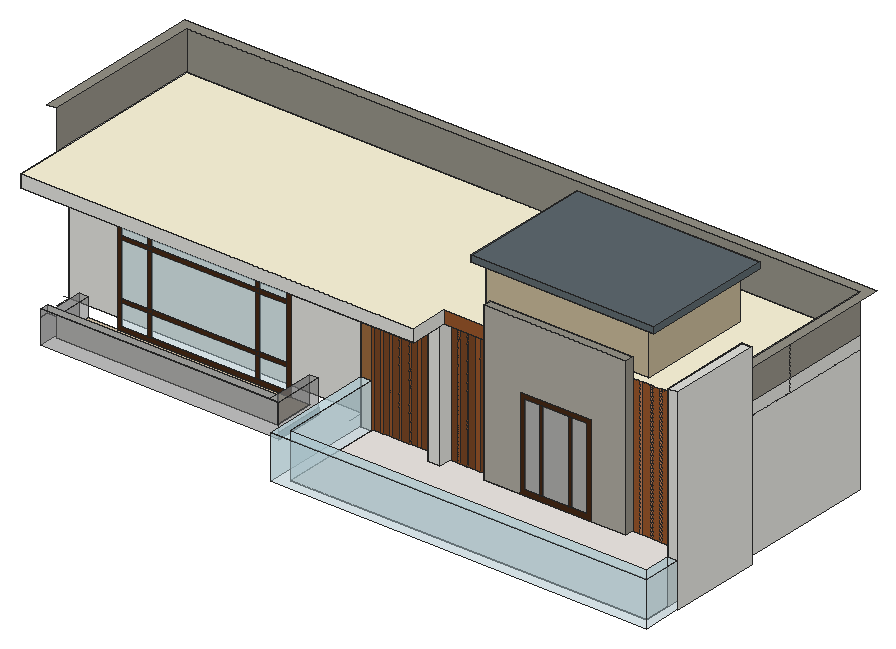
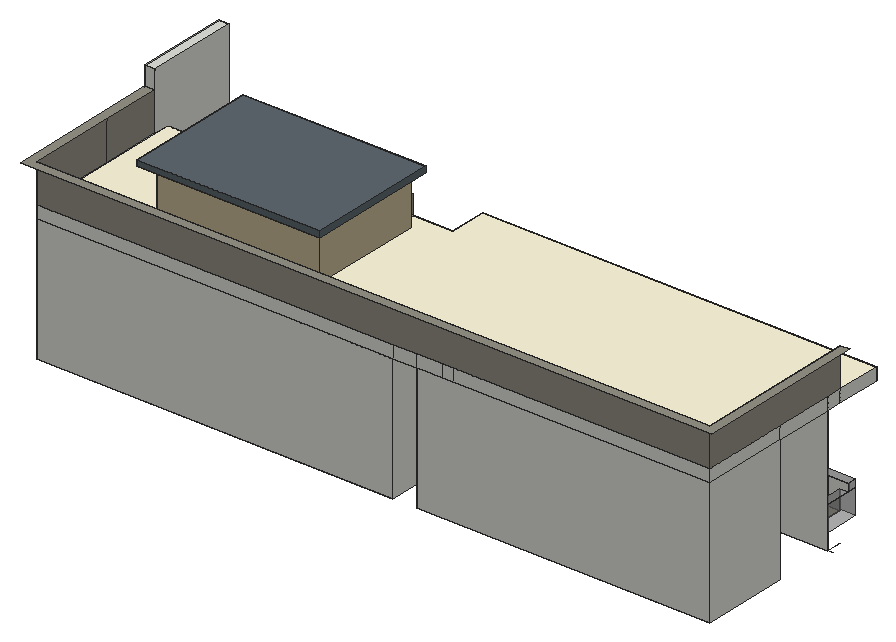
# SketchUp Ruby script. Lengths in inches.
U = 1.inch
M = Sketchup.active_model
def pt(a) = Geom::Point3d.new(a.map { |v| v * U })
def face(e, loops, mat)
  f = e.add_face(loops[0].map { |a| pt(a) })
  loops[1..].each { |l| e.add_face(l.map { |a| pt(a) }).erase! }
  f.material = f.back_material = mat if mat
  f
end
# faces: each face lists its corners as indices into pts; further lists are holes
def faces(e, pts, list, mat = nil) = list.each { |f| face(e, (f[0].is_a?(Array) ? f : [f]).map { |l| l.map { |i| pts[i] } }, mat) }
# xy, xz, yz: faces in a plane at the given z, y or x. An outline is a flat list of corners, or four numbers for a rectangle; further outlines are holes
def ring(l) = l.size == 4 ? [[l[0], l[1]], [l[2], l[1]], [l[2], l[3]], [l[0], l[3]]] : l.each_slice(2).to_a
def flat(e, list, mat, &to3) = list.each { |f| face(e, (f[0].is_a?(Array) ? f : [f]).map { |l| ring(l).map { |u, v| to3.(u, v) } }, mat) }
def xy(e, z, list, mat = nil) = flat(e, list, mat) { |x, y| [x, y, z] }
def xz(e, y, list, mat = nil) = flat(e, list, mat) { |x, z| [x, y, z] }
def yz(e, x, list, mat = nil) = flat(e, list, mat) { |y, z| [x, y, z] }
def lines(e, pts, list) = list.each { |a, b| e.add_line(pt(pts[a]), pt(pts[b])) }
# prism: a flat outline (further loops are holes) pulled along v
def prism(e, loops, v, mat = nil)
  f = face(e, loops, mat); d = Geom::Vector3d.new(v.map { |x| x * U })
  f.pushpull(f.normal.samedirection?(d) ? d.length : -d.length)
end
def box(e, o, s, mat = nil) = prism(e, [[o, [o[0] + s[0], o[1], o[2]], [o[0] + s[0], o[1] + s[1], o[2]], [o[0], o[1] + s[1], o[2]]]], [0, 0, s[2]], mat)
def at(x, y, z, deg = 0) = Geom::Transformation.translation(pt([x, y, z])) * Geom::Transformation.rotation(ORIGIN, Z_AXIS, deg.degrees)
def axes(o, x, y, z) = Geom::Transformation.new([*x, 0, *y, 0, *z, 0, *pt(o).to_a, 1])
def part(name) = M.definitions.add(name)
# library, detail: a bought-in or finely detailed component or shape, given as its bounding box
def library(name, o, s) = part(name).tap { |d| box(d.entities, o, s) }
def detail(e, o, s) = box(e.add_group.entities, o, s)
def put(e, d, t, mat = nil) = e.add_instance(d, t).tap { |i| i.material = mat if mat }
def group(e, t, mat = nil) = e.add_group.tap { |g| g.transformation = t; g.material = mat if mat }.entities
root = M.entities
M.materials.add("[0051_Cornsilk]").color = [255, 248, 220]
M.materials.add("[Color M00]").color = [255, 255, 255]
M.materials.add("[Formica Graystone]").color = [149, 146, 135]
M.materials.add("[Formica Speckled Grey]").color = [94, 105, 111]
M.materials.add("[Quartz Light Brown]").color = [199, 184, 152]
M.materials.add("[Rough Square Concrete Block]").color = [175, 171, 161]
M.materials.add("[Tile Various Tan]").color = [214, 196, 169]
M.materials.add("[Translucent Glass Gray]").color = [128, 128, 128]
M.materials["[Translucent Glass Gray]"].alpha = 0.5
M.materials.add("[Translucent Glass Safety]").color = [204, 235, 244]
M.materials["[Translucent Glass Safety]"].alpha = 0.5
M.materials.add("[Translucent Glass Safety]1").color = [204, 235, 244]
M.materials["[Translucent Glass Safety]1"].alpha = 0.5
M.materials.add("[White Square Tile]").color = [240, 234, 230]
M.materials.add("[Wood Bamboo]").color = [177, 105, 43]
M.materials.add("[Wood Cherry Original]").color = [152, 86, 42]
M.materials.add("[Wood Floor]").color = [155, 105, 61]
M.materials.add("[Wood Veneer 01]").color = [71, 41, 22]
M.materials.add("[Wood Veneer 01]1").color = [120, 70, 37]
M.materials.add("[Wood Veneer 02]").color = [190, 128, 91]
xy(root,141,[[374.25,169.4,386.5,181.59],[424.63,173.96,560.8,181.59],[302.6,179.4,312.93,181.59],[312.93,190.8,653.71,337.49],[9,253.79,289.99,337.49]])
xy(root,141,[[40.13,142.8,251.69,181.59]],"[Tile Various Tan]")
xy(root,141,[[312.93,82.84,653.71,82.84,653.71,181.59,560.8,181.59,560.8,173.96,424.63,173.96,424.63,181.59,386.5,181.59,386.5,169.4,374.25,169.4,374.25,181.59,312.93,181.59]],"[White Square Tile]")
xy(root,159.5,[[31.69,142.8,40.13,181.59]],"[Translucent Glass Gray]")
xy(root,166.97,[[31.69,133.78,251.69,142.8],[251.69,133.78,260.31,181.59]],"[Translucent Glass Gray]")
xy(root,183.75,[[302.6,70.96,662.71,70.96,662.71,108.47,653.71,108.47,653.71,82.84,312.93,82.84,312.93,179.4,302.6,179.4]],"[Translucent Glass Safety]1")
xy(root,261,[[21.23,155.71,20.74,155.74,20.27,155.82,19.8,155.94,19.35,156.11,18.91,156.33,18.51,156.6,18.13,156.9,17.79,157.25,17.48,157.62,17.22,158.03,17,158.46,16.83,158.91,16.7,159.38,16.625,159.86,16.6,160.34,16.625,160.82,16.7,161.3,16.83,161.77,17,162.22,17.22,162.65,17.48,163.06,17.79,163.43,18.13,163.78,18.51,164.08,18.91,164.35,19.35,164.56,19.8,164.74,20.27,164.86,20.74,164.9375,21.23,164.96,21.71,164.9375,22.1875,164.86,22.66,164.74,23.11,164.56,23.54,164.35,23.95,164.08,24.32,163.78,24.66,163.43,24.97,163.06,25.23,162.65,25.45,162.22,25.625,161.77,25.75,161.3,25.83,160.82,25.85,160.34,25.83,159.86,25.75,159.38,25.625,158.91,25.45,158.46,25.23,158.03,24.97,157.62,24.66,157.25,24.32,156.9,23.95,156.6,23.54,156.33,23.11,156.11,22.66,155.94,22.1875,155.82,21.71,155.74],[63.73,155.71,63.24,155.74,62.77,155.82,62.3,155.94,61.85,156.11,61.41,156.33,61.01,156.6,60.63,156.9,60.29,157.25,59.98,157.62,59.72,158.03,59.5,158.46,59.33,158.91,59.2,159.38,59.125,159.86,59.1,160.34,59.125,160.82,59.2,161.3,59.33,161.77,59.5,162.22,59.72,162.65,59.98,163.06,60.29,163.43,60.63,163.78,61.01,164.08,61.41,164.35,61.85,164.56,62.3,164.74,62.77,164.86,63.24,164.9375,63.73,164.96,64.21,164.9375,64.6875,164.86,65.16,164.74,65.61,164.56,66.04,164.35,66.45,164.08,66.82,163.78,67.16,163.43,67.47,163.06,67.73,162.65,67.95,162.22,68.125,161.77,68.25,161.3,68.33,160.82,68.35,160.34,68.33,159.86,68.25,159.38,68.125,158.91,67.95,158.46,67.73,158.03,67.47,157.62,67.16,157.25,66.82,156.9,66.45,156.6,66.04,156.33,65.61,156.11,65.16,155.94,64.6875,155.82,64.21,155.74],[115.79,155.71,115.31,155.74,114.83,155.82,114.36,155.94,113.91,156.11,113.48,156.33,113.07,156.6,112.69,156.9,112.35,157.25,112.05,157.62,111.78,158.03,111.5625,158.46,111.39,158.91,111.27,159.38,111.1875,159.86,111.16,160.34,111.1875,160.82,111.27,161.3,111.39,161.77,111.5625,162.22,111.78,162.65,112.05,163.06,112.35,163.43,112.69,163.78,113.07,164.08,113.48,164.35,113.91,164.56,114.36,164.74,114.83,164.86,115.31,164.9375,115.79,164.96,116.27,164.9375,116.75,164.86,117.22,164.74,117.67,164.56,118.1,164.35,118.51,164.08,118.88,163.78,119.23,163.43,119.53,163.06,119.79,162.65,120.01,162.22,120.1875,161.77,120.3125,161.3,120.39,160.82,120.41,160.34,120.39,159.86,120.3125,159.38,120.1875,158.91,120.01,158.46,119.79,158.03,119.53,157.62,119.23,157.25,118.88,156.9,118.51,156.6,118.1,156.33,117.67,156.11,117.22,155.94,116.75,155.82,116.27,155.74],[172.66,155.71,172.18,155.74,171.7,155.82,171.23,155.94,170.78,156.11,170.35,156.33,169.95,156.6,169.57,156.9,169.23,157.25,168.92,157.62,168.66,158.03,168.4375,158.46,168.27,158.91,168.14,159.38,168.0625,159.86,168.04,160.34,168.0625,160.82,168.14,161.3,168.27,161.77,168.4375,162.22,168.66,162.65,168.92,163.06,169.23,163.43,169.57,163.78,169.95,164.08,170.35,164.35,170.78,164.56,171.23,164.74,171.7,164.86,172.18,164.9375,172.66,164.96,173.15,164.9375,173.625,164.86,174.09,164.74,174.55,164.56,174.98,164.35,175.38,164.08,175.76,163.78,176.1,163.43,176.41,163.06,176.67,162.65,176.89,162.22,177.0625,161.77,177.1875,161.3,177.26,160.82,177.29,160.34,177.26,159.86,177.1875,159.38,177.0625,158.91,176.89,158.46,176.67,158.03,176.41,157.62,176.1,157.25,175.76,156.9,175.38,156.6,174.98,156.33,174.55,156.11,174.09,155.94,173.625,155.82,173.15,155.74],[221.35,155.71,220.87,155.74,220.39,155.82,219.92,155.94,219.47,156.11,219.04,156.33,218.63,156.6,218.26,156.9,217.91,157.25,217.61,157.62,217.35,158.03,217.125,158.46,216.95,158.91,216.83,159.38,216.75,159.86,216.73,160.34,216.75,160.82,216.83,161.3,216.95,161.77,217.125,162.22,217.35,162.65,217.61,163.06,217.91,163.43,218.26,163.78,218.63,164.08,219.04,164.35,219.47,164.56,219.92,164.74,220.39,164.86,220.87,164.9375,221.35,164.96,221.84,164.9375,222.3125,164.86,222.78,164.74,223.23,164.56,223.66,164.35,224.07,164.08,224.45,163.78,224.79,163.43,225.09,163.06,225.36,162.65,225.58,162.22,225.75,161.77,225.875,161.3,225.95,160.82,225.98,160.34,225.95,159.86,225.875,159.38,225.75,158.91,225.58,158.46,225.36,158.03,225.09,157.62,224.79,157.25,224.45,156.9,224.07,156.6,223.66,156.33,223.23,156.11,222.78,155.94,222.3125,155.82,221.84,155.74],
  [280.54,155.71,280.06,155.74,279.58,155.82,279.11,155.94,278.66,156.11,278.23,156.33,277.82,156.6,277.44,156.9,277.1,157.25,276.8,157.62,276.53,158.03,276.3125,158.46,276.14,158.91,276.02,159.38,275.9375,159.86,275.91,160.34,275.9375,160.82,276.02,161.3,276.14,161.77,276.3125,162.22,276.53,162.65,276.8,163.06,277.1,163.43,277.44,163.78,277.82,164.08,278.23,164.35,278.66,164.56,279.11,164.74,279.58,164.86,280.06,164.9375,280.54,164.96,281.02,164.9375,281.5,164.86,281.97,164.74,282.42,164.56,282.85,164.35,283.26,164.08,283.63,163.78,283.98,163.43,284.28,163.06,284.54,162.65,284.76,162.22,284.9375,161.77,285.0625,161.3,285.14,160.82,285.16,160.34,285.14,159.86,285.0625,159.38,284.9375,158.91,284.76,158.46,284.54,158.03,284.28,157.62,283.98,157.25,283.63,156.9,283.26,156.6,282.85,156.33,282.42,156.11,281.97,155.94,281.5,155.82,281.02,155.74],[317.16,155.71,316.68,155.74,316.2,155.82,315.73,155.94,315.28,156.11,314.85,156.33,314.45,156.6,314.07,156.9,313.73,157.25,313.42,157.62,313.16,158.03,312.9375,158.46,312.77,158.91,312.64,159.38,312.5625,159.86,312.54,160.34,312.5625,160.82,312.64,161.3,312.77,161.77,312.9375,162.22,313.16,162.65,313.42,163.06,313.73,163.43,314.07,163.78,314.45,164.08,314.85,164.35,315.28,164.56,315.73,164.74,316.2,164.86,316.68,164.9375,317.16,164.96,317.65,164.9375,318.125,164.86,318.59,164.74,319.05,164.56,319.48,164.35,319.88,164.08,320.26,163.78,320.6,163.43,320.91,163.06,321.17,162.65,321.39,162.22,321.5625,161.77,321.6875,161.3,321.76,160.82,321.79,160.34,321.76,159.86,321.6875,159.38,321.5625,158.91,321.39,158.46,321.17,158.03,320.91,157.62,320.6,157.25,320.26,156.9,319.88,156.6,319.48,156.33,319.05,156.11,318.59,155.94,318.125,155.82,317.65,155.74],[358.29,155.71,357.81,155.74,357.33,155.82,356.86,155.94,356.41,156.11,355.98,156.33,355.57,156.6,355.19,156.9,354.85,157.25,354.55,157.62,354.28,158.03,354.0625,158.46,353.89,158.91,353.77,159.38,353.6875,159.86,353.66,160.34,353.6875,160.82,353.77,161.3,353.89,161.77,354.0625,162.22,354.28,162.65,354.55,163.06,354.85,163.43,355.19,163.78,355.57,164.08,355.98,164.35,356.41,164.56,356.86,164.74,357.33,164.86,357.81,164.9375,358.29,164.96,358.77,164.9375,359.25,164.86,359.72,164.74,360.17,164.56,360.6,164.35,361.01,164.08,361.38,163.78,361.73,163.43,362.03,163.06,362.29,162.65,362.51,162.22,362.6875,161.77,362.8125,161.3,362.89,160.82,362.91,160.34,362.89,159.86,362.8125,159.38,362.6875,158.91,362.51,158.46,362.29,158.03,362.03,157.62,361.73,157.25,361.38,156.9,361.01,156.6,360.6,156.33,360.17,156.11,359.72,155.94,359.25,155.82,358.77,155.74],[374.25,169.4,386.5,181.59],[302.6,179.4,312.93,181.59],
  [312.93,190.8,653.71,196.16],[9,196.16,312.93,253.79],[312.93,196.16,653.71,253.79],[9,253.79,289.99,337.49],[289.99,253.79,312.93,337.49],
  [312.93,253.79,653.71,337.49]])
xy(root,261,[[[9,138.15,9,181.59,302.6,181.59,302.6,179.4,312.93,179.4,312.93,181.59,374.25,181.59,374.25,169.4,386.5,169.4,386.5,138.15],[21.23,155.71,21.71,155.74,22.1875,155.82,22.66,155.94,23.11,156.11,23.54,156.33,23.95,156.6,24.32,156.9,24.66,157.25,24.97,157.62,25.23,158.03,25.45,158.46,25.625,158.91,25.75,159.38,25.83,159.86,25.85,160.34,25.83,160.82,25.75,161.3,25.625,161.77,25.45,162.22,25.23,162.65,24.97,163.06,24.66,163.43,24.32,163.78,23.95,164.08,23.54,164.35,23.11,164.56,22.66,164.74,22.1875,164.86,21.71,164.9375,21.23,164.96,20.74,164.9375,20.27,164.86,19.8,164.74,19.35,164.56,18.91,164.35,18.51,164.08,18.13,163.78,17.79,163.43,17.48,163.06,17.22,162.65,17,162.22,16.83,161.77,16.7,161.3,16.625,160.82,16.6,160.34,16.625,159.86,16.7,159.38,16.83,158.91,17,158.46,17.22,158.03,17.48,157.62,17.79,157.25,18.13,156.9,18.51,156.6,18.91,156.33,19.35,156.11,19.8,155.94,20.27,155.82,20.74,155.74],[317.16,155.71,317.65,155.74,318.125,155.82,318.59,155.94,319.05,156.11,319.48,156.33,319.88,156.6,320.26,156.9,320.6,157.25,320.91,157.62,321.17,158.03,321.39,158.46,321.5625,158.91,321.6875,159.38,321.76,159.86,321.79,160.34,321.76,160.82,321.6875,161.3,321.5625,161.77,321.39,162.22,321.17,162.65,320.91,163.06,320.6,163.43,320.26,163.78,319.88,164.08,319.48,164.35,319.05,164.56,318.59,164.74,318.125,164.86,317.65,164.9375,317.16,164.96,316.68,164.9375,316.2,164.86,315.73,164.74,315.28,164.56,314.85,164.35,314.45,164.08,314.07,163.78,313.73,163.43,313.42,163.06,313.16,162.65,312.9375,162.22,312.77,161.77,312.64,161.3,312.5625,160.82,312.54,160.34,312.5625,159.86,312.64,159.38,312.77,158.91,312.9375,158.46,313.16,158.03,313.42,157.62,313.73,157.25,314.07,156.9,314.45,156.6,314.85,156.33,315.28,156.11,315.73,155.94,316.2,155.82,316.68,155.74],[63.73,155.71,64.21,155.74,64.6875,155.82,65.16,155.94,65.61,156.11,66.04,156.33,66.45,156.6,66.82,156.9,67.16,157.25,67.47,157.62,67.73,158.03,67.95,158.46,68.125,158.91,68.25,159.38,68.33,159.86,68.35,160.34,68.33,160.82,68.25,161.3,68.125,161.77,67.95,162.22,67.73,162.65,67.47,163.06,67.16,163.43,66.82,163.78,66.45,164.08,66.04,164.35,65.61,164.56,65.16,164.74,64.6875,164.86,64.21,164.9375,63.73,164.96,63.24,164.9375,62.77,164.86,62.3,164.74,61.85,164.56,61.41,164.35,61.01,164.08,60.63,163.78,60.29,163.43,59.98,163.06,59.72,162.65,59.5,162.22,59.33,161.77,59.2,161.3,59.125,160.82,59.1,160.34,59.125,159.86,59.2,159.38,59.33,158.91,59.5,158.46,59.72,158.03,59.98,157.62,60.29,157.25,60.63,156.9,61.01,156.6,61.41,156.33,61.85,156.11,62.3,155.94,62.77,155.82,63.24,155.74],[280.54,155.71,281.02,155.74,281.5,155.82,281.97,155.94,282.42,156.11,282.85,156.33,283.26,156.6,283.63,156.9,283.98,157.25,284.28,157.62,284.54,158.03,284.76,158.46,284.9375,158.91,285.0625,159.38,285.14,159.86,285.16,160.34,285.14,160.82,285.0625,161.3,284.9375,161.77,284.76,162.22,284.54,162.65,284.28,163.06,283.98,163.43,283.63,163.78,283.26,164.08,282.85,164.35,282.42,164.56,281.97,164.74,281.5,164.86,281.02,164.9375,280.54,164.96,280.06,164.9375,279.58,164.86,279.11,164.74,278.66,164.56,278.23,164.35,277.82,164.08,277.44,163.78,277.1,163.43,276.8,163.06,276.53,162.65,276.3125,162.22,276.14,161.77,276.02,161.3,275.9375,160.82,275.91,160.34,275.9375,159.86,276.02,159.38,276.14,158.91,276.3125,158.46,276.53,158.03,276.8,157.62,277.1,157.25,277.44,156.9,277.82,156.6,278.23,156.33,278.66,156.11,279.11,155.94,279.58,155.82,280.06,155.74],[115.79,155.71,116.27,155.74,116.75,155.82,117.22,155.94,117.67,156.11,118.1,156.33,118.51,156.6,118.88,156.9,119.23,157.25,119.53,157.62,119.79,158.03,120.01,158.46,120.1875,158.91,120.3125,159.38,120.39,159.86,120.41,160.34,120.39,160.82,120.3125,161.3,120.1875,161.77,120.01,162.22,119.79,162.65,119.53,163.06,119.23,163.43,118.88,163.78,118.51,164.08,118.1,164.35,117.67,164.56,117.22,164.74,116.75,164.86,116.27,164.9375,115.79,164.96,115.31,164.9375,114.83,164.86,114.36,164.74,113.91,164.56,113.48,164.35,113.07,164.08,112.69,163.78,112.35,163.43,112.05,163.06,111.78,162.65,111.5625,162.22,111.39,161.77,111.27,161.3,111.1875,160.82,111.16,160.34,111.1875,159.86,111.27,159.38,111.39,158.91,111.5625,158.46,111.78,158.03,112.05,157.62,112.35,157.25,112.69,156.9,113.07,156.6,113.48,156.33,113.91,156.11,114.36,155.94,114.83,155.82,115.31,155.74],[221.35,155.71,221.84,155.74,222.3125,155.82,222.78,155.94,223.23,156.11,223.66,156.33,224.07,156.6,224.45,156.9,224.79,157.25,225.09,157.62,225.36,158.03,225.58,158.46,225.75,158.91,225.875,159.38,225.95,159.86,225.98,160.34,225.95,160.82,225.875,161.3,225.75,161.77,225.58,162.22,225.36,162.65,225.09,163.06,224.79,163.43,224.45,163.78,224.07,164.08,223.66,164.35,223.23,164.56,222.78,164.74,222.3125,164.86,221.84,164.9375,221.35,164.96,220.87,164.9375,220.39,164.86,219.92,164.74,219.47,164.56,219.04,164.35,218.63,164.08,218.26,163.78,217.91,163.43,217.61,163.06,217.35,162.65,217.125,162.22,216.95,161.77,216.83,161.3,216.75,160.82,216.73,160.34,216.75,159.86,216.83,159.38,216.95,158.91,217.125,158.46,217.35,158.03,217.61,157.62,217.91,157.25,218.26,156.9,218.63,156.6,219.04,156.33,219.47,156.11,219.92,155.94,220.39,155.82,220.87,155.74],[172.66,155.71,173.15,155.74,173.625,155.82,174.09,155.94,174.55,156.11,174.98,156.33,175.38,156.6,175.76,156.9,176.1,157.25,176.41,157.62,176.67,158.03,176.89,158.46,177.0625,158.91,177.1875,159.38,177.26,159.86,177.29,160.34,177.26,160.82,177.1875,161.3,177.0625,161.77,176.89,162.22,176.67,162.65,176.41,163.06,176.1,163.43,175.76,163.78,175.38,164.08,174.98,164.35,174.55,164.56,174.09,164.74,173.625,164.86,173.15,164.9375,172.66,164.96,172.18,164.9375,171.7,164.86,171.23,164.74,170.78,164.56,170.35,164.35,169.95,164.08,169.57,163.78,169.23,163.43,168.92,163.06,168.66,162.65,168.4375,162.22,168.27,161.77,168.14,161.3,168.0625,160.82,168.04,160.34,168.0625,159.86,168.14,159.38,168.27,158.91,168.4375,158.46,168.66,158.03,168.92,157.62,169.23,157.25,169.57,156.9,169.95,156.6,170.35,156.33,170.78,156.11,171.23,155.94,171.7,155.82,172.18,155.74],[358.29,155.71,358.77,155.74,359.25,155.82,359.72,155.94,360.17,156.11,360.6,156.33,361.01,156.6,361.38,156.9,361.73,157.25,362.03,157.62,362.29,158.03,362.51,158.46,362.6875,158.91,362.8125,159.38,362.89,159.86,362.91,160.34,362.89,160.82,362.8125,161.3,362.6875,161.77,362.51,162.22,362.29,162.65,362.03,163.06,361.73,163.43,361.38,163.78,361.01,164.08,360.6,164.35,360.17,164.56,359.72,164.74,359.25,164.86,358.77,164.9375,358.29,164.96,357.81,164.9375,357.33,164.86,356.86,164.74,356.41,164.56,355.98,164.35,355.57,164.08,355.19,163.78,354.85,163.43,354.55,163.06,354.28,162.65,354.0625,162.22,353.89,161.77,353.77,161.3,353.6875,160.82,353.66,160.34,353.6875,159.86,353.77,159.38,353.89,158.91,354.0625,158.46,354.28,158.03,354.55,157.62,354.85,157.25,355.19,156.9,355.57,156.6,355.98,156.33,356.41,156.11,356.86,155.94,357.33,155.82,357.81,155.74]]],"[Wood Bamboo]")
xy(root,261,[[386.5,173.96,424.63,181.59]],"[Wood Cherry Original]")
xy(root,273,[[[9,138.15,386.5,138.15,386.5,173.96,424.63,173.96,424.63,181.59,653.71,181.59,653.71,337.49,9,337.49],[414.15,189.53,570.65,298.28]]],"[0051_Cornsilk]")
xy(root,291,[[424.63,173.96,560.8,181.59]],"[Formica Graystone]")
xy(root,310.4375,[[0,181.59,9,181.59,9,337.49,653.71,337.49,653.71,196.8125,662.71,196.8125,662.71,346.49,0,346.49]],"[Formica Graystone]")
xy(root,318.625,[[407.09,180.78,581.84,189.53],[407.09,189.53,414.15,307.53],[414.15,189.53,570.65,298.28],[570.65,189.53,581.84,307.53],[414.15,298.28,570.65,307.53]])
xy(root,324.375,[[407.09,180.78,581.84,307.53]],"[Formica Speckled Grey]")
xy(root,328.3125,[[653.71,108.47,662.71,196.8125]])
xz(root,70.96,[[302.6,141,662.71,183.75]],"[Translucent Glass Safety]1")
xz(root,82.84,[[312.93,141,653.71,183.75]],"[Translucent Glass Safety]1")
xz(root,108.47,[[653.71,183.75,662.71,328.3125]])
xz(root,133.78,[[31.69,135,260.09,135,260.09,141,260.31,166.97,31.69,166.97]],"[Translucent Glass Gray]")
xz(root,138.15,[[9,261,386.5,273]])
xz(root,142.8,[[40.13,141,40.13,159.5,31.69,159.5,31.69,166.97,251.69,166.97,251.69,141]])
xz(root,169.4,[[374.25,141,386.5,261]])
xz(root,173.96,[[424.63,141,459.54,141,459.54,228.5625,527.66,228.5625,527.66,141,560.8,141,560.8,291,424.63,291]],"[Rough Square Concrete Block]")
xz(root,173.96,[[464.33,145.79,478.25,223.77],[480.65,145.79,506.37,223.77],[508.77,145.79,522.87,223.77]],"[Translucent Glass Gray]")
xz(root,173.96,[[386.5,261,424.63,273]],"[Wood Cherry Original]")
xz(root,173.96,[[[459.54,141,527.66,228.5625],[464.33,145.79,522.87,223.77]],[478.25,145.79,480.65,223.77],[506.37,145.79,508.77,223.77]],"[Wood Veneer 01]")
xz(root,179.4,[[302.6,141,312.93,183.75]])
xz(root,179.4,[[302.6,183.75,312.93,261]],"[Wood Floor]")
xz(root,180.78,[[407.09,318.625,581.84,324.375]],"[Formica Speckled Grey]")
xz(root,181.59,[[302.6,141,312.93,261],[374.25,141,386.5,261],[424.63,141,560.8,261],[424.63,261,560.8,273],[424.63,273,560.8,291]])
xz(root,181.59,[[386.5,141,386.57,261]],"[Color M00]")
xz(root,181.59,[[71.91,145.08,96.9,165.54],[100.71,145.08,199.91,165.54],[203.5,145.08,229.7,165.54],[71.91,169.15,96.9,219.6],[100.71,169.15,199.91,219.6],
  [203.5,169.15,229.7,219.6],[71.91,223.22,96.9,245.05],[100.71,223.22,199.91,245.05],[203.5,223.22,229.7,245.05]],"[Translucent Glass Safety]")
xz(root,181.59,[[319.79,141,321.62,261],[328.48,141,330.5,261],[337.36,141,339.62,261],[346.48,141,348.31,261],[355.17,141,357.85,261],
  [364.71,141,367.39,261],[393.43,141,395.64,261],[402.5,141,403.57,261],[410.43,141,414.51,261],[421.37,141,424.63,261],
  [560.8,141,568.2,273],[570.68,141,578.08,273],[580.05,141,587.45,273],[589.43,141,596.83,273],[598.8,141,606.2,273],
  [608.18,141,615.58,273],[617.55,141,624.95,273],[626.93,141,634.33,273],[636.3,141,643.7,273],[646.31,141,653.71,273]],"[Wood Cherry Original]")
xz(root,181.59,[[[67.84,141,233.77,249.125],[71.91,145.08,229.7,245.05]],[96.9,145.08,100.71,165.54],[199.91,145.08,203.5,165.54],[71.91,165.54,96.9,169.15],[96.9,165.54,100.71,169.15],
  [100.71,165.54,199.91,169.15],[199.91,165.54,203.5,169.15],[203.5,165.54,229.7,169.15],[96.9,169.15,100.71,219.6],[199.91,169.15,203.5,219.6],
  [71.91,219.6,96.9,223.22],[96.9,219.6,100.71,223.22],[100.71,219.6,199.91,223.22],[199.91,219.6,203.5,223.22],[203.5,219.6,229.7,223.22],
  [96.9,223.22,100.71,245.05],[199.91,223.22,203.5,245.05]],"[Wood Veneer 01]")
xz(root,181.59,[[312.93,141,319.79,261],[321.62,141,328.48,261],[330.5,141,337.36,261],[339.62,141,346.48,261],[348.31,141,355.17,261],
  [357.85,141,364.71,261],[367.39,141,374.25,261],[386.57,141,393.43,261],[395.64,141,402.5,261],[403.57,141,410.43,261],
  [414.51,141,421.37,261]],"[Wood Veneer 01]1")
xz(root,181.59,[[568.2,141,570.68,273],[578.08,141,580.05,273],[587.45,141,589.43,273],[596.83,141,598.8,273],[606.2,141,608.18,273],
  [615.58,141,617.55,273],[624.95,141,626.93,273],[634.33,141,636.3,273],[643.7,141,646.31,273]],"[Wood Veneer 02]")
xz(root,189.53,[[414.15,273,570.65,318.625]],"[Quartz Light Brown]")
xz(root,190.8,[[312.93,141,653.71,261]])
xz(root,196.16,[[9,141,289.99,261]])
xz(root,196.8125,[[653.71,310.4375,662.71,328.3125]])
xz(root,253.79,[[9,141,289.99,261]])
xz(root,298.28,[[414.15,273,570.65,318.625]],"[Quartz Light Brown]")
xz(root,307.53,[[407.09,318.625,581.84,324.375]],"[Formica Speckled Grey]")
xz(root,337.49,[[9,141,289.99,261],[312.93,141,653.71,261],[9,261,254.94,273],[254.94,261,265.25,273],[265.25,261,289.99,273],
  [289.99,261,312.93,273],[312.93,261,653.71,273]])
xz(root,337.49,[[9,273,653.71,310.4375]],"[Formica Graystone]")
yz(root,9,[[196.16,141,196.8125,261],[253.79,141,337.49,261],[138.15,261,181.59,273],[181.59,261,196.16,273],[196.16,261,196.8125,273],
  [196.8125,261,253.79,273],[253.79,261,337.49,273]])
yz(root,9,[[181.59,273,337.49,310.4375]],"[Formica Graystone]")
yz(root,31.69,[[133.78,135,181.59,159.5],[133.78,159.5,142.8,166.97]],"[Translucent Glass Gray]")
yz(root,40.13,[[142.8,141,181.59,159.5]],"[Translucent Glass Gray]")
yz(root,251.69,[[142.8,141,181.59,166.97]],"[Translucent Glass Gray]")
yz(root,260.09,[[133.78,135,181.59,141]],"[Formica Speckled Grey]")
yz(root,289.99,[[253.79,141,337.49,261]])
yz(root,302.6,[[70.96,141,179.4,183.75]],"[Translucent Glass Safety]1")
yz(root,302.6,[[179.4,141,181.59,261]],"[Wood Veneer 02]")
yz(root,312.93,[[190.8,141,337.49,261]])
yz(root,312.93,[[82.84,141,179.4,183.75]],"[Translucent Glass Safety]1")
yz(root,312.93,[[179.4,141,181.59,261]],"[Wood Cherry Original]")
yz(root,374.25,[[169.4,141,181.59,261]])
yz(root,386.5,[[169.4,141,181.59,261],[138.15,261,173.96,273]])
yz(root,407.09,[[180.78,318.625,307.53,324.375]],"[Formica Speckled Grey]")
yz(root,414.15,[[189.53,273,298.28,318.625]],"[Quartz Light Brown]")
yz(root,424.63,[[173.96,261,181.59,273]])
yz(root,424.63,[[173.96,273,181.59,291]],"[Formica Graystone]")
yz(root,424.63,[[173.96,141,181.59,261]],"[Wood Cherry Original]")
yz(root,560.8,[[173.96,141,181.59,291]],"[Formica Graystone]")
yz(root,570.65,[[189.53,273,298.28,318.625]],"[Quartz Light Brown]")
yz(root,581.84,[[180.78,318.625,307.53,324.375]],"[Formica Speckled Grey]")
yz(root,653.71,[[108.47,141,108.47,328.3125,196.16,328.3125,196.16,273,181.59,273,181.59,141],[190.8,141,196.8125,261],[196.8125,141,337.49,261],[181.59,261,190.8,273],[190.8,261,196.16,273],
  [196.16,261,196.8125,273],[196.8125,261,253.79,273],[253.79,261,337.49,273],[196.16,273,196.8125,328.3125]])
yz(root,653.71,[[196.8125,273,253.79,310.4375],[253.79,273,337.49,310.4375]],"[Formica Graystone]")
yz(root,653.71,[[82.84,141,108.47,183.75]],"[Translucent Glass Safety]1")
yz(root,662.71,[[108.47,141,196.8125,328.3125]])
yz(root,662.71,[[70.96,141,108.47,183.75]],"[Translucent Glass Safety]1")
p = [[260.09,181.59,141],[260.31,181.59,166.97],[260.31,133.78,166.97],[260.09,133.78,141],[9,181.59,141],[9,196.16,141],
  [289.99,181.59,141],[289.99,196.16,141],[4.12,196.16,141]]
faces(root,p,[[0,1,2,3]],"[Translucent Glass Gray]")
lines(root,p,[[4,5],[6,7],[5,8]])
